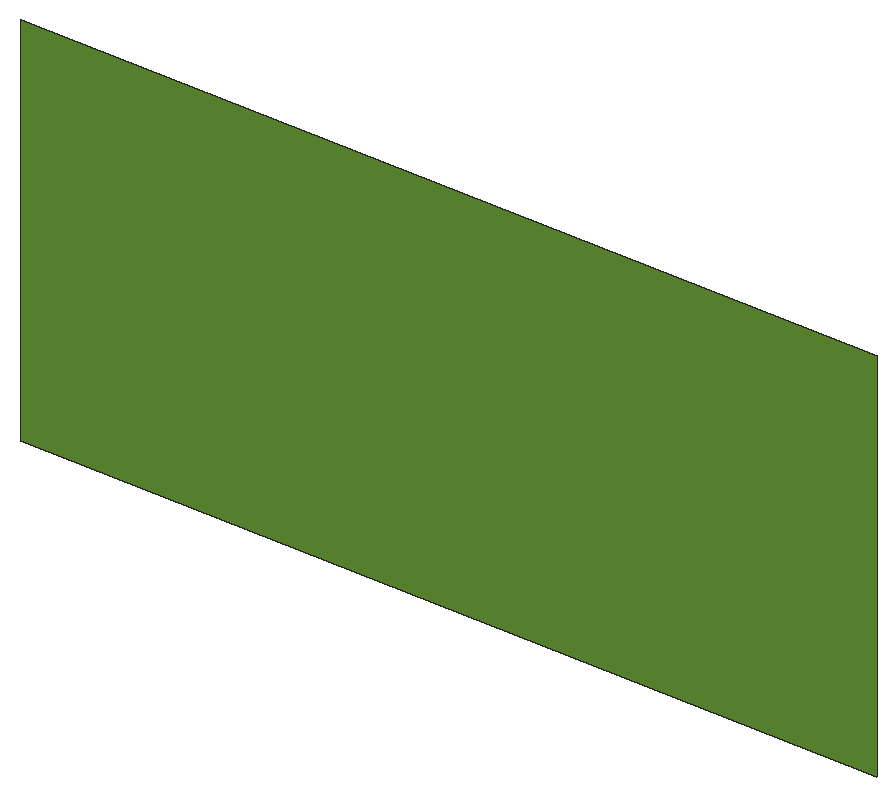
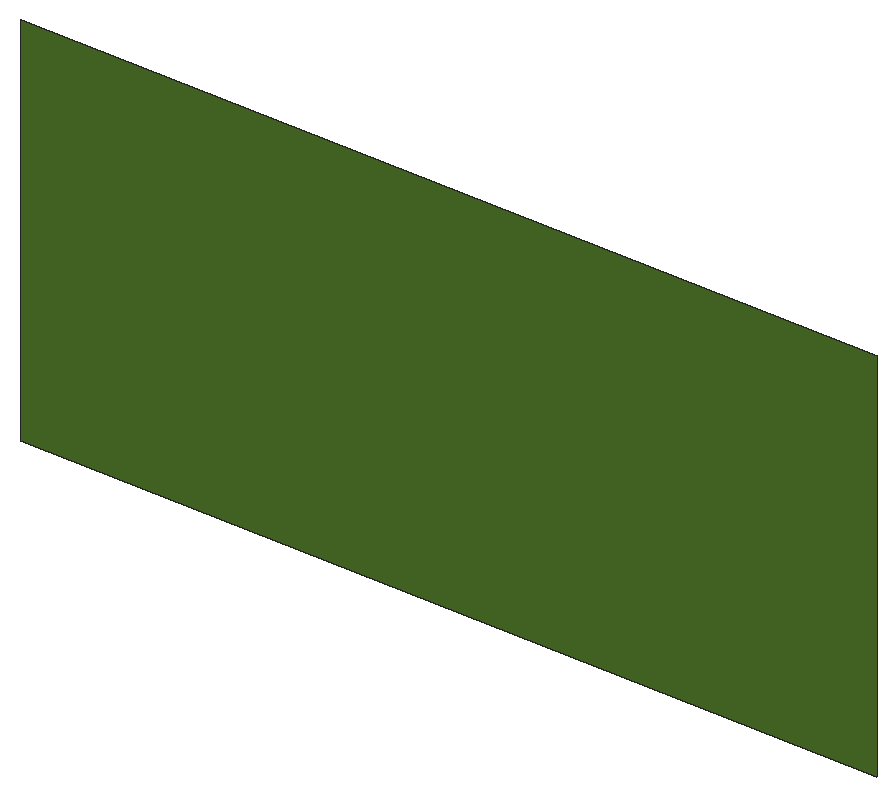
# SketchUp Ruby script. Lengths in inches.
U = 1.inch
M = Sketchup.active_model
def pt(a) = Geom::Point3d.new(a.map { |v| v * U })
def face(e, loops, mat)
  f = e.add_face(loops[0].map { |a| pt(a) })
  loops[1..].each { |l| e.add_face(l.map { |a| pt(a) }).erase! }
  f.material = f.back_material = mat if mat
  f
end
# faces: each face lists its corners as indices into pts; further lists are holes
def faces(e, pts, list, mat = nil) = list.each { |f| face(e, (f[0].is_a?(Array) ? f : [f]).map { |l| l.map { |i| pts[i] } }, mat) }
# xy, xz, yz: faces in a plane at the given z, y or x. An outline is a flat list of corners, or four numbers for a rectangle; further outlines are holes
def ring(l) = l.size == 4 ? [[l[0], l[1]], [l[2], l[1]], [l[2], l[3]], [l[0], l[3]]] : l.each_slice(2).to_a
def flat(e, list, mat, &to3) = list.each { |f| face(e, (f[0].is_a?(Array) ? f : [f]).map { |l| ring(l).map { |u, v| to3.(u, v) } }, mat) }
def xy(e, z, list, mat = nil) = flat(e, list, mat) { |x, y| [x, y, z] }
def xz(e, y, list, mat = nil) = flat(e, list, mat) { |x, z| [x, y, z] }
def yz(e, x, list, mat = nil) = flat(e, list, mat) { |y, z| [x, y, z] }
def lines(e, pts, list) = list.each { |a, b| e.add_line(pt(pts[a]), pt(pts[b])) }
# prism: a flat outline (further loops are holes) pulled along v
def prism(e, loops, v, mat = nil)
  f = face(e, loops, mat); d = Geom::Vector3d.new(v.map { |x| x * U })
  f.pushpull(f.normal.samedirection?(d) ? d.length : -d.length)
end
def box(e, o, s, mat = nil) = prism(e, [[o, [o[0] + s[0], o[1], o[2]], [o[0] + s[0], o[1] + s[1], o[2]], [o[0], o[1] + s[1], o[2]]]], [0, 0, s[2]], mat)
def at(x, y, z, deg = 0) = Geom::Transformation.translation(pt([x, y, z])) * Geom::Transformation.rotation(ORIGIN, Z_AXIS, deg.degrees)
def axes(o, x, y, z) = Geom::Transformation.new([*x, 0, *y, 0, *z, 0, *pt(o).to_a, 1])
def part(name) = M.definitions.add(name)
# library, detail: a bought-in or finely detailed component or shape, given as its bounding box
def library(name, o, s) = part(name).tap { |d| box(d.entities, o, s) }
def detail(e, o, s) = box(e.add_group.entities, o, s)
def put(e, d, t, mat = nil) = e.add_instance(d, t).tap { |i| i.material = mat if mat }
def group(e, t, mat = nil) = e.add_group.tap { |g| g.transformation = t; g.material = mat if mat }.entities
root = M.entities
M.materials.add("[Grass Dark Green]").color = [106, 157, 55]
xz(root,80.93,[[25.26,9,42.01,16.375]],"[Grass Dark Green]")
